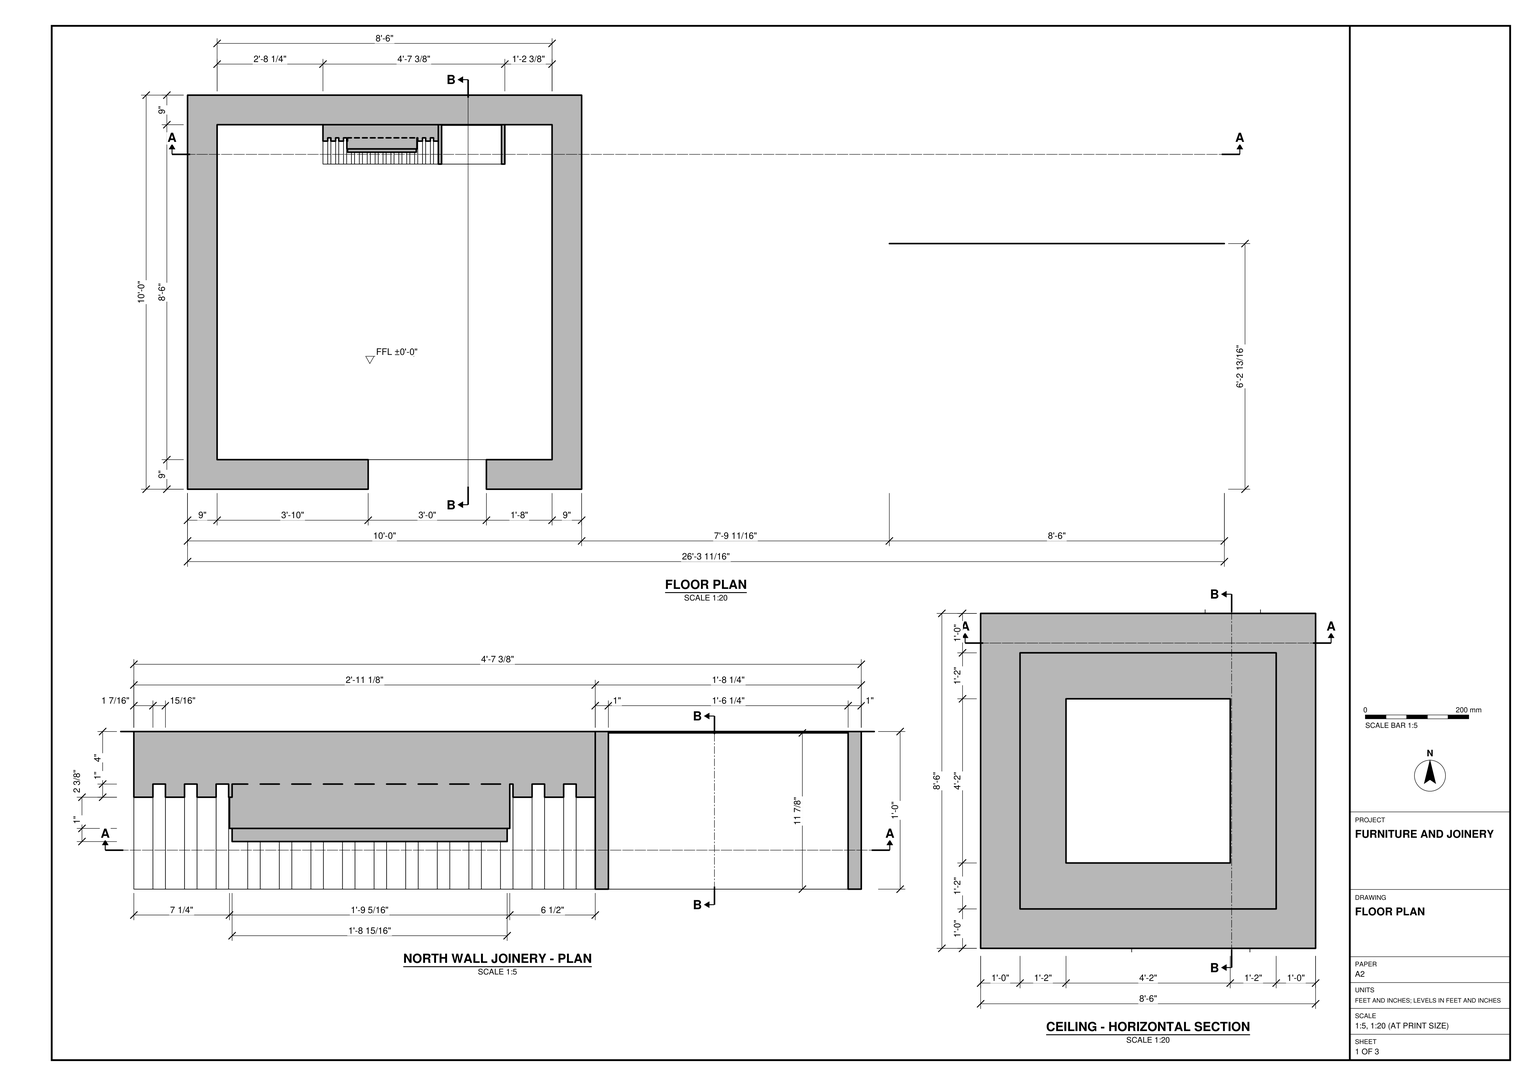
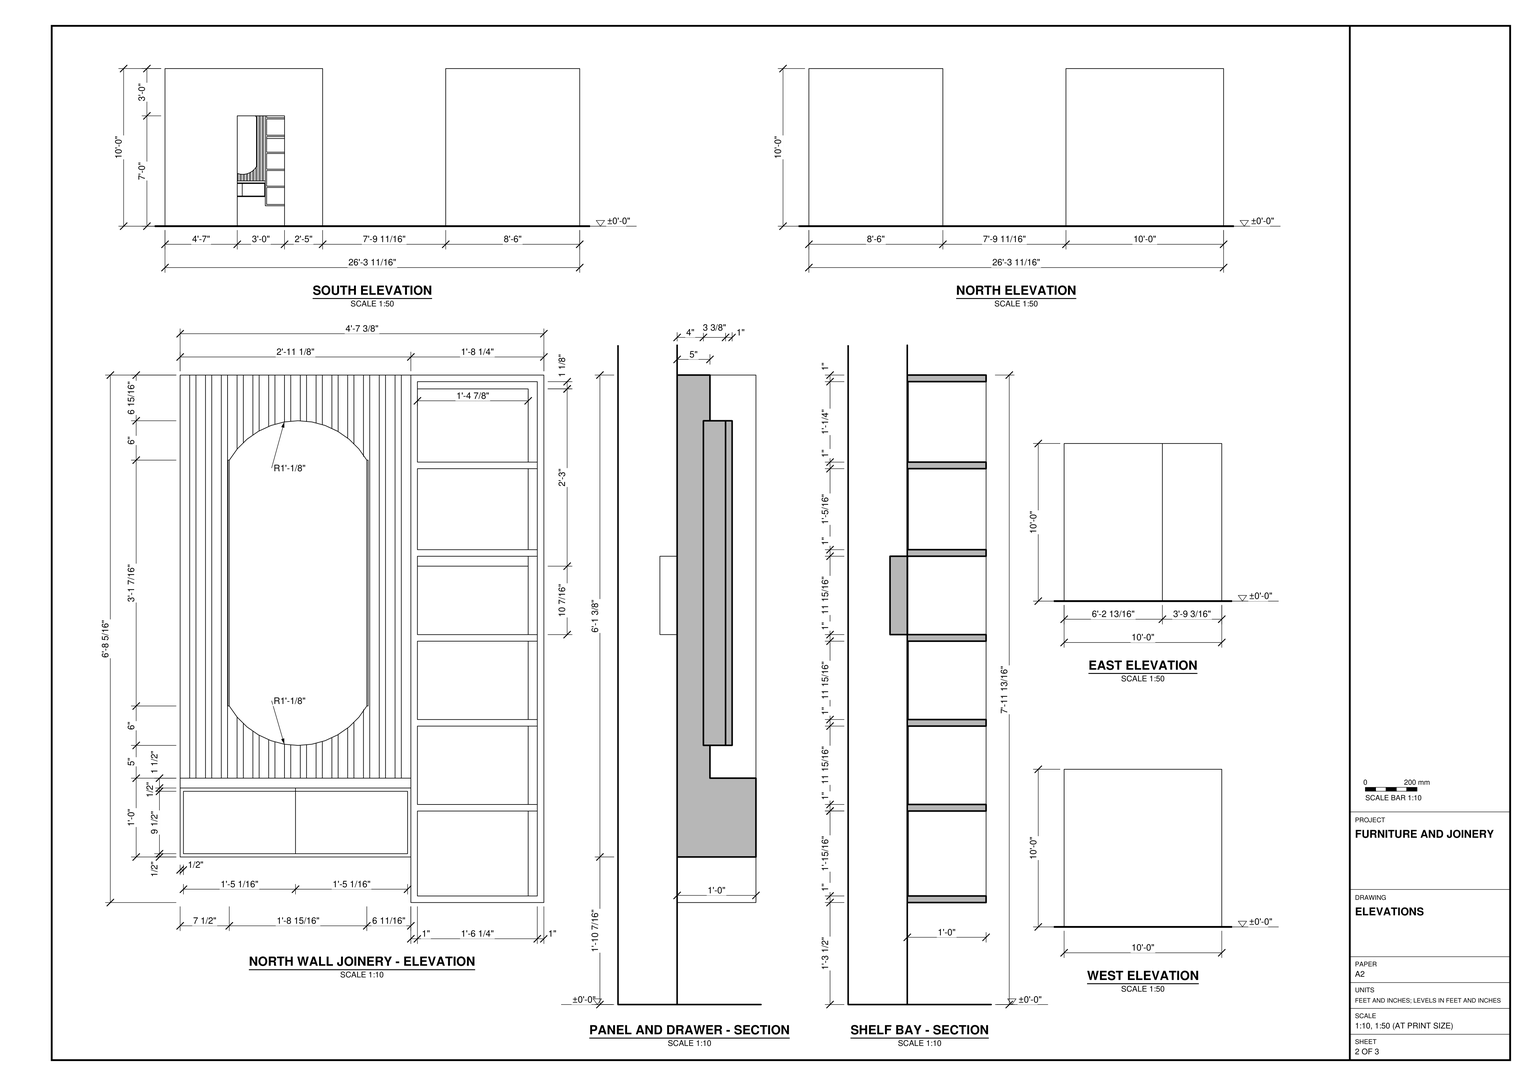
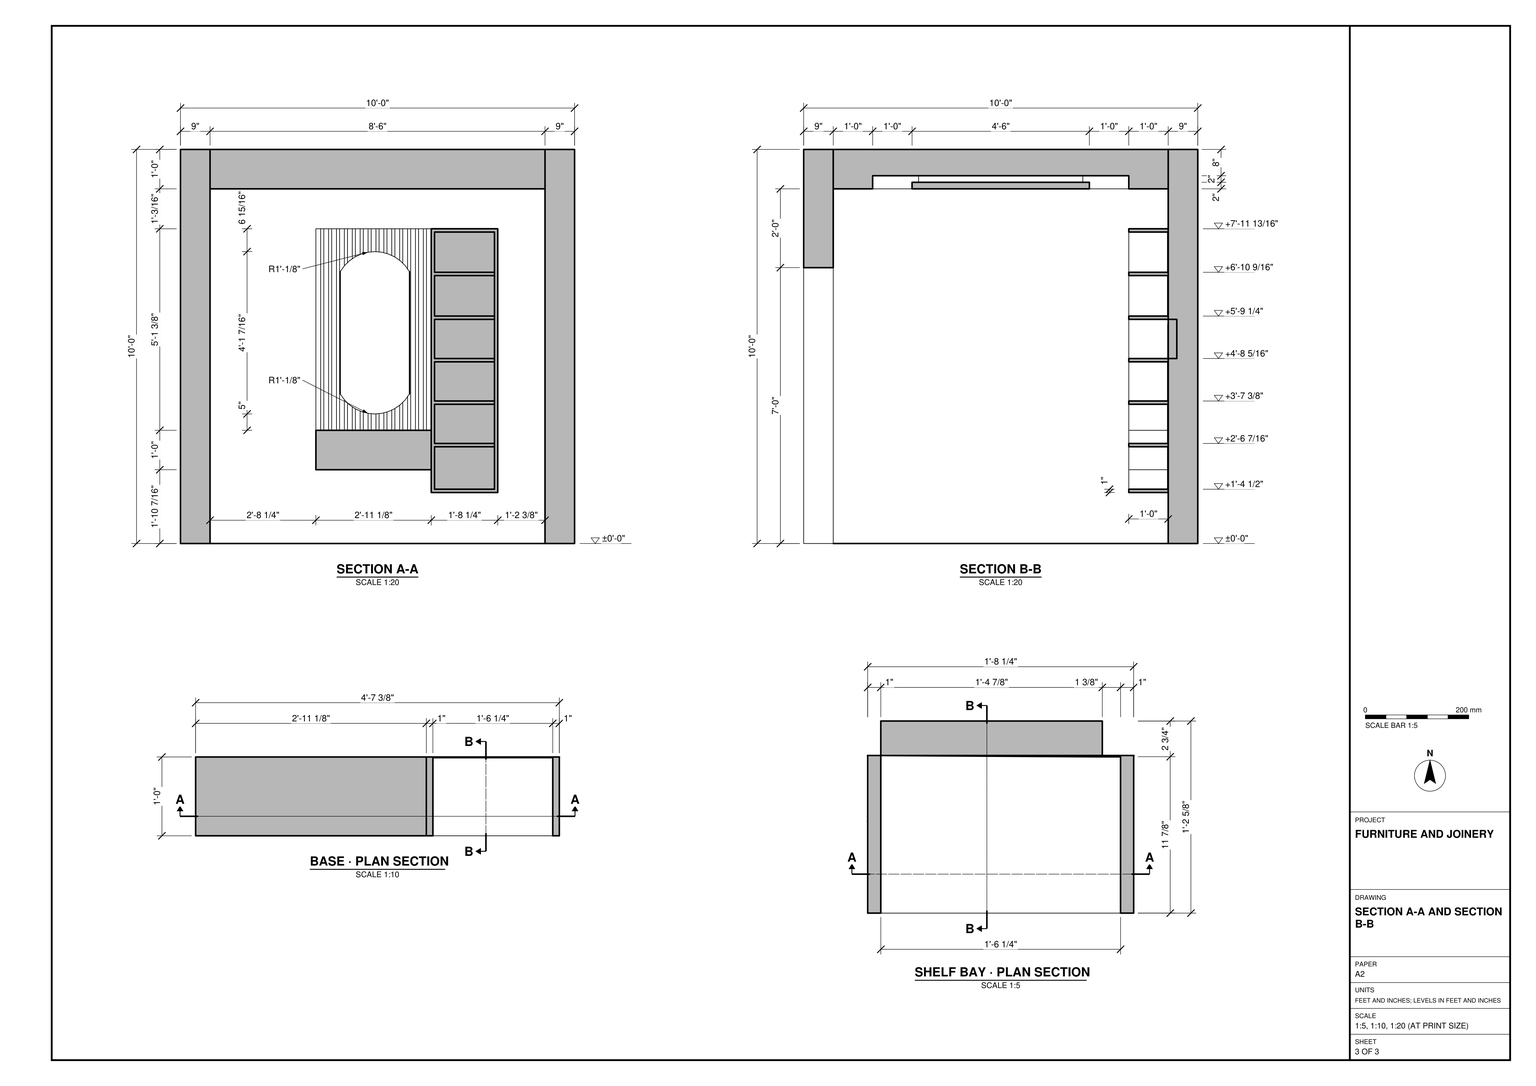
Build the room and its fitted joinery in SketchUp from task_files/diagram_01.pdf. Work in feet and inches. The overall model is 26'-3 11/16" along X, 10'-0" along Y and 10'-0" high, with a single finished floor level at ±0'-0". The room itself is 10'-0" square externally. The remaining X extent includes the gap and the separate upright surface shown east of the room; use the floor plan to locate that surface and the elevations to set its height.

Build the 9" perimeter walls and leave the offset doorway in the south wall, with the wall continuing above the opening. Form the stepped ceiling using the ceiling horizontal section for the square outlines and section B-B for their depths.

Fit the joinery against the inside of the north wall. Use the detailed elevation to lay out the wide, vertically slatted mirror panel on the left, the suspended drawer unit beneath it and the narrower open shelf bay on the right. Model the mirror with straight sides and curved ends. Align the tops of the two bays, but extend the shelving below the drawer unit as shown. Use the detailed sections to set the projections, shelf thicknesses and mounting heights.

Keep the shell elements and each joinery or furniture piece in separate groups or components, and use components for repeated parts. Any decor or loose items shown may use suitable library components. Save one SketchUp model as output_files/room_and_its_north_wall_mirror_and_shelf_unit.skp.

# SketchUp Ruby script. Lengths in inches.
U = 1.inch
M = Sketchup.active_model
def pt(a) = Geom::Point3d.new(a.map { |v| v * U })
def face(e, loops, mat)
  f = e.add_face(loops[0].map { |a| pt(a) })
  loops[1..].each { |l| e.add_face(l.map { |a| pt(a) }).erase! }
  f.material = f.back_material = mat if mat
  f
end
# faces: each face lists its corners as indices into pts; further lists are holes
def faces(e, pts, list, mat = nil) = list.each { |f| face(e, (f[0].is_a?(Array) ? f : [f]).map { |l| l.map { |i| pts[i] } }, mat) }
# xy, xz, yz: faces in a plane at the given z, y or x. An outline is a flat list of corners, or four numbers for a rectangle; further outlines are holes
def ring(l) = l.size == 4 ? [[l[0], l[1]], [l[2], l[1]], [l[2], l[3]], [l[0], l[3]]] : l.each_slice(2).to_a
def flat(e, list, mat, &to3) = list.each { |f| face(e, (f[0].is_a?(Array) ? f : [f]).map { |l| ring(l).map { |u, v| to3.(u, v) } }, mat) }
def xy(e, z, list, mat = nil) = flat(e, list, mat) { |x, y| [x, y, z] }
def xz(e, y, list, mat = nil) = flat(e, list, mat) { |x, z| [x, y, z] }
def yz(e, x, list, mat = nil) = flat(e, list, mat) { |y, z| [x, y, z] }
def lines(e, pts, list) = list.each { |a, b| e.add_line(pt(pts[a]), pt(pts[b])) }
# prism: a flat outline (further loops are holes) pulled along v
def prism(e, loops, v, mat = nil)
  f = face(e, loops, mat); d = Geom::Vector3d.new(v.map { |x| x * U })
  f.pushpull(f.normal.samedirection?(d) ? d.length : -d.length)
end
def box(e, o, s, mat = nil) = prism(e, [[o, [o[0] + s[0], o[1], o[2]], [o[0] + s[0], o[1] + s[1], o[2]], [o[0], o[1] + s[1], o[2]]]], [0, 0, s[2]], mat)
def at(x, y, z, deg = 0) = Geom::Transformation.translation(pt([x, y, z])) * Geom::Transformation.rotation(ORIGIN, Z_AXIS, deg.degrees)
def axes(o, x, y, z) = Geom::Transformation.new([*x, 0, *y, 0, *z, 0, *pt(o).to_a, 1])
def part(name) = M.definitions.add(name)
# library, detail: a bought-in or finely detailed component or shape, given as its bounding box
def library(name, o, s) = part(name).tap { |d| box(d.entities, o, s) }
def detail(e, o, s) = box(e.add_group.entities, o, s)
def put(e, d, t, mat = nil) = e.add_instance(d, t).tap { |i| i.material = mat if mat }
def group(e, t, mat = nil) = e.add_group.tap { |g| g.transformation = t; g.material = mat if mat }.entities
root = M.entities
M.materials.add("[Color A01]").color = [255, 204, 204]
M.materials.add("[Color A01]1").color = [255, 204, 204]
M.materials.add("[Color A01]2").color = [255, 247, 239]
M.materials.add("[Color M01]").color = [226, 226, 226]
M.materials.add("[Color M05]").color = [114, 114, 114]
M.materials.add("[Mirror 01]").color = [185, 185, 185]
M.materials.add("[Wood Bamboo]").color = [177, 105, 43]
M.materials.add("[Wood Veneer 01]").color = [120, 70, 37]
c1 = part("Component\#1")
xz(c1.entities,0,[[0,0,102,120]])
xy(root,0,[[0,0,0,120,120,120,120,0,91,0,91,9,111,9,111,111,9,111,9,9,55,9,55,0],[9,9,111,111]])
xy(root,84,[[55,0,91,9]])
xy(root,120,[[[0,0,120,120],[9,9,111,111]]])
xz(root,0,[[0,0,55,0,55,84,91,84,91,0,120,0,120,120,0,120]])
xz(root,9,[[9,0,9,120,111,120,111,0,91,0,91,84,55,84,55,0]])
xz(root,111,[[9,0,111,120]])
xz(root,120,[[0,0,120,120]])
yz(root,0,[[0,0,120,120]])
yz(root,9,[[9,0,111,120]])
yz(root,55,[[0,0,9,84]])
yz(root,76.36,[[99,34.47,106,95.84]],"[Wood Bamboo]")
yz(root,91,[[0,0,9,84]])
yz(root,111,[[9,0,111,120]])
yz(root,120,[[0,0,120,120]])
g1 = group(root,at(213.7,74.8,0))
xy(g1,15.53,[[-137.34,24.2,-117.09,36.2]],"[Wood Veneer 01]")
xy(g1,16.53,[[-119.48,36.1,-118.09,36.2]],"[Color A01]1")
xy(g1,16.53,[[-136.34,24.2,-118.09,36.1],[-136.34,36.1,-119.48,36.2]],"[Wood Veneer 01]")
xy(g1,22.47,[[-172.47,24.2,-137.34,36.2]])
xy(g1,29.46,[[-119.48,36.1,-118.09,36.2]],"[Color A01]1")
xy(g1,29.46,[[-136.34,24.2,-118.09,36.1],[-136.34,36.1,-119.48,36.2]],"[Wood Veneer 01]")
xy(g1,30.46,[[-119.48,36.1,-118.09,36.2]],"[Color A01]1")
xy(g1,30.46,[[-136.34,24.2,-118.09,36.1],[-136.34,36.1,-119.48,36.2]],"[Wood Veneer 01]")
xy(g1,34.47,[[-172.47,24.2,-171.01,31.2],[-171.01,24.2,-170.06,32.2],[-170.06,24.2,-168.61,31.2],[-168.61,24.2,-167.65,32.2],[-167.65,24.2,-166.2,31.2],
  [-166.2,24.2,-165.25,32.2],[-165.25,24.2,-163.8,31.2],[-163.8,24.2,-162.84,32.2],[-162.84,24.2,-161.39,31.2],[-161.39,24.2,-160.44,32.2],
  [-160.44,24.2,-158.99,31.2],[-158.99,24.2,-158.03,32.2],[-158.03,24.2,-156.58,31.2],[-156.58,24.2,-155.63,32.2],[-155.63,24.2,-154.18,31.2],
  [-154.18,24.2,-153.22,32.2],[-153.22,24.2,-151.77,31.2],[-151.77,24.2,-150.82,32.2],[-150.82,24.2,-149.37,31.2],[-149.37,24.2,-148.41,32.2],
  [-148.41,24.2,-146.96,31.2],[-146.96,24.2,-146.01,32.2],[-146.01,24.2,-144.56,31.2],[-144.56,24.2,-143.6,32.2],[-143.6,24.2,-142.15,31.2],
  [-142.15,24.2,-141.2,32.2],[-141.2,24.2,-139.75,31.2],[-139.75,24.2,-138.79,32.2],[-138.79,24.2,-137.34,31.2]])
xy(g1,39.64,[[-156.61,31.2,-156.58,32.2]])
xy(g1,42.4,[[-119.48,36.1,-118.09,36.2]],"[Color A01]1")
xy(g1,42.4,[[-136.34,24.2,-118.09,36.1],[-136.34,36.1,-119.48,36.2]],"[Wood Veneer 01]")
xy(g1,43.4,[[-119.48,36.1,-118.09,36.2]],"[Color A01]1")
xy(g1,43.4,[[-136.34,24.2,-118.09,36.1],[-136.34,36.1,-119.48,36.2]],"[Wood Veneer 01]")
xy(g1,45.46,[[-165.19,28.83,-164.99,31.2],[-144.05,28.83,-143.85,32.2]],"[Color A01]")
xy(g1,55.33,[[-119.48,36.1,-118.09,36.2]],"[Color A01]1")
xy(g1,55.33,[[-136.34,24.2,-118.09,36.1],[-136.34,36.1,-119.48,36.2]],"[Wood Veneer 01]")
xy(g1,56.33,[[-119.48,36.1,-119.48,36.2,-136.34,36.2]])
xy(g1,56.33,[[-119.48,36.1,-118.09,36.2]],"[Color A01]1")
xy(g1,56.33,[[-136.34,24.2,-118.09,24.2,-118.09,36.1,-119.48,36.1,-136.34,36.2],[-136.34,36.2,-119.48,38.83]],"[Wood Veneer 01]")
xy(g1,68.26,[[-119.48,36.1,-118.09,36.2]],"[Color A01]1")
xy(g1,68.26,[[-136.34,24.2,-136.34,36.2,-119.48,36.2,-119.48,36.1,-118.09,36.1,-118.09,24.2],[-136.34,36.2,-119.48,38.83]],"[Wood Veneer 01]")
xy(g1,69.26,[[-119.48,36.1,-118.09,36.2]],"[Color A01]1")
xy(g1,69.26,[[-136.34,24.2,-118.09,36.1],[-136.34,36.1,-119.48,36.2]],"[Wood Veneer 01]")
xy(g1,81.59,[[-119.48,36.1,-118.09,36.2]],"[Color A01]1")
xy(g1,81.59,[[-136.34,24.2,-118.09,36.1],[-136.34,36.1,-119.48,36.2]],"[Wood Veneer 01]")
xy(g1,82.59,[[-119.48,36.1,-118.09,36.2]],"[Color A01]1")
xy(g1,82.59,[[-136.34,24.2,-118.09,36.1],[-136.34,36.1,-119.48,36.2]],"[Wood Veneer 01]")
xy(g1,82.89,[[-165.19,28.83,-164.99,31.2],[-144.05,28.83,-143.85,32.2]],"[Color A01]")
xy(g1,88.71,[[-156.61,31.2,-156.58,32.2]])
xy(g1,94.84,[[-136.34,36.1,-118.09,36.2]],"[Color A01]1")
xy(g1,94.84,[[-136.34,24.2,-118.09,36.1]],"[Wood Veneer 01]")
xy(g1,95.84,[[-172.47,31.2,-171.01,31.2,-171.01,32.2,-170.06,32.2,-170.06,31.2,-168.61,31.2,-168.61,32.2,-167.65,32.2,-167.65,31.2,-166.2,31.2,-166.2,32.2,-165.25,32.2,-165.25,31.2,-163.8,31.2,-163.8,32.2,-162.84,32.2,-162.84,31.2,-161.39,31.2,-161.39,32.2,-160.44,32.2,-160.44,31.2,-158.99,31.2,-158.99,32.2,-158.03,32.2,-158.03,31.2,-156.58,31.2,-156.58,32.2,-155.63,32.2,-155.63,31.2,-154.18,31.2,-154.18,32.2,-153.22,32.2,-153.22,31.2,-151.77,31.2,-151.77,32.2,-150.82,32.2,-150.82,31.2,-149.37,31.2,-149.37,32.2,-148.41,32.2,-148.41,31.2,-146.96,31.2,-146.96,32.2,-146.01,32.2,-146.01,31.2,-144.56,31.2,-144.56,32.2,-143.6,32.2,-143.6,31.2,-142.15,31.2,-142.15,32.2,-141.2,32.2,-141.2,31.2,-139.75,31.2,-139.75,32.2,-138.79,32.2,-138.79,31.2,-137.34,31.2,-137.34,36.2,-172.47,36.2]])
xy(g1,95.84,[[-137.34,24.2,-117.09,36.2]],"[Wood Veneer 01]")
xz(g1,24.2,[[-172.47,22.47,-137.34,22.47,-137.34,32.97,-154.9,32.97,-154.9,32.47,-137.84,32.47,-137.84,22.97,-171.97,22.97,-171.97,32.47,-154.9,32.47,-154.9,32.97,-172.47,32.97],[-171.97,22.97,-154.9,32.47],[-154.9,22.97,-137.84,32.47]])
xz(g1,24.2,[[-172.47,32.97,-137.34,34.47]],"[Color M05]")
xz(g1,24.2,[[[-137.34,15.53,-117.09,95.84],[-136.34,16.53,-136.34,29.46,-118.09,29.46,-118.09,30.46,-136.34,30.46,-136.34,42.4,-118.09,42.4,-118.09,43.4,-136.34,43.4,-136.34,55.33,-118.09,55.33,-118.09,56.33,-136.34,56.33,-136.34,68.26,-118.09,68.26,-118.09,69.26,-136.34,69.26,-136.34,81.59,-118.09,81.59,-118.09,82.59,-136.34,82.59,-136.34,94.84,-118.09,94.84,-118.09,16.53]]],"[Wood Veneer 01]")
xz(g1,27.83,[[-154.52,39.46,-152.42,39.64,-150.39,40.18,-148.48,41.0625,-146.76,42.26,-145.26,43.74,-144.05,45.46,-144.05,82.89,-145.26,84.61,-146.76,86.09,-148.48,87.29,-150.39,88.17,-152.42,88.71,-154.52,88.89,-156.61,88.71,-158.64,88.17,-160.55,87.29,-162.28,86.09,-163.77,84.61,-164.99,82.89,-164.99,45.46,-163.77,43.74,-162.28,42.26,-160.55,41.0625,-158.64,40.18,-156.61,39.64]],"[Mirror 01]")
xz(g1,28.83,[[-154.52,39.46,-156.61,39.64,-158.64,40.18,-160.55,41.0625,-162.28,42.26,-163.77,43.74,-164.99,45.46,-164.99,82.89,-163.77,84.61,-162.28,86.09,-160.55,87.29,-158.64,88.17,-156.61,88.71,-154.52,88.89,-152.42,88.71,-150.39,88.17,-148.48,87.29,-146.76,86.09,-145.26,84.61,-144.05,82.89,-144.05,45.46,-145.26,43.74,-146.76,42.26,-148.48,41.0625,-150.39,40.18,-152.42,39.64]])
xz(g1,28.83,[[-165.19,45.46,-164.99,82.89],[-144.05,45.46,-143.85,82.89]],"[Color A01]")
xz(g1,31.2,[[-172.47,34.47,-171.01,95.84],[-170.06,34.47,-168.61,95.84],[-167.65,34.47,-166.2,95.84],[-165.25,34.47,-163.8,34.47,-163.8,43.78,-164.99,45.46,-165.19,45.46,-165.19,82.89,-164.99,82.89,-163.8,84.57,-163.8,95.84,-165.25,95.84],[-162.84,34.47,-161.39,34.47,-161.39,41.65,-162.28,42.26,-162.84,42.83],
  [-160.44,34.47,-158.99,34.47,-158.99,40.34,-160.44,41.01],[-158.03,34.47,-156.58,34.47,-156.58,39.64,-156.61,39.64,-158.03,40.02],[-155.63,34.47,-154.18,34.47,-154.18,39.49,-154.52,39.46,-155.63,39.55],[-153.22,34.47,-151.77,34.47,-151.77,39.8125,-152.42,39.64,-153.22,39.57],[-150.82,34.47,-149.37,34.47,-149.37,40.65,-150.39,40.18,-150.82,40.07],
  [-148.41,34.47,-146.96,34.47,-146.96,42.12,-148.41,41.11],[-146.01,34.47,-144.56,34.47,-144.56,44.74,-145.26,43.74,-146.01,43],[-143.6,34.47,-142.15,95.84],[-141.2,34.47,-139.75,95.84],[-138.79,34.47,-137.34,95.84],
  [-144.56,83.61,-144.56,95.84,-146.01,95.84,-146.01,85.35,-145.26,84.61],[-162.84,85.52,-162.28,86.09,-161.39,86.7,-161.39,95.84,-162.84,95.84],[-146.96,86.23,-146.96,95.84,-148.41,95.84,-148.41,87.24],[-160.44,87.34,-158.99,88.01,-158.99,95.84,-160.44,95.84],[-149.37,87.7,-149.37,95.84,-150.82,95.84,-150.82,88.28,-150.39,88.17],
  [-158.03,88.33,-156.61,88.71,-156.58,88.71,-156.58,95.84,-158.03,95.84],[-151.77,88.54,-151.77,95.84,-153.22,95.84,-153.22,88.78,-152.42,88.71],[-155.63,88.8,-154.52,88.89,-154.18,88.86,-154.18,95.84,-155.63,95.84]])
xz(g1,31.2,[[-165.19,45.46,-164.99,82.89]],"[Color A01]")
xz(g1,32.2,[[-171.01,34.47,-170.06,95.84],[-168.61,34.47,-167.65,95.84],[-166.2,34.47,-165.25,95.84],[-163.8,34.47,-162.84,34.47,-162.84,42.83,-163.77,43.74,-163.8,43.78],[-161.39,34.47,-160.44,34.47,-160.44,41.01,-160.55,41.0625,-161.39,41.65],
  [-158.99,34.47,-158.03,34.47,-158.03,40.02,-158.64,40.18,-158.99,40.34],[-156.58,34.47,-155.63,34.47,-155.63,39.55,-156.58,39.64],[-154.18,34.47,-153.22,34.47,-153.22,39.57,-154.18,39.49],[-151.77,34.47,-150.82,34.47,-150.82,40.07,-151.77,39.8125],[-149.37,34.47,-148.41,34.47,-148.41,41.11,-148.48,41.0625,-149.37,40.65],
  [-146.96,34.47,-146.01,34.47,-146.01,43,-146.76,42.26,-146.96,42.12],[-144.56,34.47,-143.6,34.47,-143.6,95.84,-144.56,95.84,-144.56,83.61,-144.05,82.89,-143.85,82.89,-143.85,45.46,-144.05,45.46,-144.56,44.74],[-142.15,34.47,-141.2,95.84],[-139.75,34.47,-138.79,95.84],[-154.52,39.46,-154.18,39.49,-154.18,88.86,-154.52,88.89,-155.63,88.8,-155.63,39.55],
  [-153.22,39.57,-152.42,39.64,-151.77,39.8125,-151.77,88.54,-152.42,88.71,-153.22,88.78],[-156.61,39.64,-156.58,39.64,-156.58,88.71,-156.61,88.71,-158.03,88.33,-158.03,40.02],[-150.82,40.07,-150.39,40.18,-149.37,40.65,-149.37,87.7,-150.39,88.17,-150.82,88.28],[-158.99,40.34,-158.99,88.01,-160.44,87.34,-160.44,41.01],[-148.41,41.11,-146.96,42.12,-146.96,86.23,-148.41,87.24],
  [-161.39,41.65,-161.39,86.7,-162.28,86.09,-162.84,85.52,-162.84,42.83,-162.28,42.26],[-146.01,43,-145.26,43.74,-144.56,44.74,-144.56,83.61,-145.26,84.61,-146.01,85.35],[-163.8,43.78,-163.8,84.57,-164.99,82.89,-164.99,45.46],[-163.8,84.57,-163.77,84.61,-162.84,85.52,-162.84,95.84,-163.8,95.84],[-146.01,85.35,-146.01,95.84,-146.96,95.84,-146.96,86.23,-146.76,86.09],
  [-161.39,86.7,-160.55,87.29,-160.44,87.34,-160.44,95.84,-161.39,95.84],[-148.41,87.24,-148.41,95.84,-149.37,95.84,-149.37,87.7,-148.48,87.29],[-158.99,88.01,-158.64,88.17,-158.03,88.33,-158.03,95.84,-158.99,95.84],[-150.82,88.28,-150.82,95.84,-151.77,95.84,-151.77,88.54],[-156.58,88.71,-155.63,88.8,-155.63,95.84,-156.58,95.84],
  [-153.22,88.78,-153.22,95.84,-154.18,95.84,-154.18,88.86]])
xz(g1,36.1,[[-119.48,16.53,-118.09,29.46],[-119.48,30.46,-118.09,42.4],[-119.48,43.4,-118.09,55.33],[-119.48,56.33,-118.09,68.26],[-119.48,69.26,-118.09,81.59],
  [-119.48,82.59,-118.09,82.59,-118.09,94.84,-136.34,94.84,-136.34,93.74,-119.48,93.74]],"[Color A01]1")
xz(g1,36.1,[[-136.34,16.53,-119.48,29.46],[-136.34,30.46,-119.48,42.4],[-136.34,43.4,-119.48,55.33],[-136.34,69.26,-119.48,81.59],[-136.34,82.59,-119.48,93.74]],"[Wood Veneer 01]")
xz(g1,36.2,[[[-137.34,15.53,-117.09,95.84],[-136.34,16.53,-118.09,16.53,-118.09,94.84,-136.34,94.84,-136.34,82.59,-118.09,82.59,-118.09,81.59,-136.34,81.59,-136.34,69.26,-118.09,69.26,-118.09,68.26,-136.34,68.26,-136.34,56.33,-118.09,56.33,-118.09,55.33,-136.34,55.33,-136.34,43.4,-118.09,43.4,-118.09,42.4,-136.34,42.4,-136.34,30.46,-118.09,30.46,-118.09,29.46,-136.34,29.46]],[-172.47,22.47,-137.34,95.84]])
xz(g1,38.83,[[-136.34,56.33,-119.48,68.26]],"[Wood Veneer 01]")
yz(g1,-172.47,[[31.2,34.47,36.2,95.84]])
yz(g1,-172.47,[[24.2,22.47,36.2,34.47]],"[Color M05]")
yz(g1,-171.01,[[31.2,34.47,32.2,95.84]])
yz(g1,-170.06,[[31.2,34.47,32.2,95.84]])
yz(g1,-168.61,[[31.2,34.47,32.2,95.84]])
yz(g1,-167.65,[[31.2,34.47,32.2,95.84]])
yz(g1,-166.2,[[31.2,34.47,32.2,95.84]])
yz(g1,-165.25,[[31.2,34.47,32.2,95.84]])
yz(g1,-165.19,[[28.83,45.46,31.2,82.89]],"[Color A01]")
yz(g1,-164.99,[[27.83,45.46,28.83,82.89],[31.2,45.46,32.2,82.89]])
yz(g1,-163.8,[[31.2,34.47,32.2,43.78],[31.2,84.57,32.2,95.84]])
yz(g1,-162.84,[[31.2,34.47,32.2,42.83],[31.2,85.52,32.2,95.84]])
yz(g1,-161.39,[[31.2,34.47,32.2,41.65],[31.2,86.7,32.2,95.84]])
yz(g1,-160.44,[[31.2,34.47,32.2,41.01],[31.2,87.34,32.2,95.84]])
yz(g1,-158.99,[[31.2,34.47,32.2,40.34],[31.2,88.01,32.2,95.84]])
yz(g1,-158.03,[[31.2,34.47,32.2,40.02],[31.2,88.33,32.2,95.84]])
yz(g1,-156.58,[[31.2,34.47,32.2,39.64],[31.2,88.71,32.2,95.84]])
yz(g1,-155.63,[[31.2,34.47,32.2,39.55],[31.2,88.8,32.2,95.84]])
yz(g1,-154.18,[[31.2,34.47,32.2,39.49],[31.2,88.86,32.2,95.84]])
yz(g1,-153.22,[[31.2,34.47,32.2,39.57],[31.2,88.78,32.2,95.84]])
yz(g1,-151.77,[[31.2,34.47,32.2,39.8125],[31.2,88.54,32.2,95.84]])
yz(g1,-150.82,[[31.2,34.47,32.2,40.07],[31.2,88.28,32.2,95.84]])
yz(g1,-149.37,[[31.2,34.47,32.2,40.65],[31.2,87.7,32.2,95.84]])
yz(g1,-148.41,[[31.2,34.47,32.2,41.11],[31.2,87.24,32.2,95.84]])
yz(g1,-146.96,[[31.2,34.47,32.2,42.12],[31.2,86.23,32.2,95.84]])
yz(g1,-146.01,[[31.2,34.47,32.2,43],[31.2,85.35,32.2,95.84]])
yz(g1,-144.56,[[31.2,34.47,32.2,44.74],[31.2,83.61,32.2,95.84]])
yz(g1,-144.05,[[27.83,45.46,28.83,82.89]])
yz(g1,-143.85,[[28.83,45.46,32.2,82.89]],"[Color A01]")
yz(g1,-143.6,[[31.2,34.47,32.2,95.84]])
yz(g1,-142.15,[[31.2,34.47,32.2,95.84]])
yz(g1,-141.2,[[31.2,34.47,32.2,95.84]])
yz(g1,-139.75,[[31.2,34.47,32.2,95.84]])
yz(g1,-138.79,[[31.2,34.47,32.2,95.84]])
yz(g1,-137.34,[[24.2,22.47,36.2,34.47],[24.2,34.47,31.2,95.84],[31.2,34.47,36.2,95.84]])
yz(g1,-137.34,[[24.2,15.53,36.2,22.47]],"[Wood Veneer 01]")
yz(g1,-136.34,[[36.1,93.74,36.2,94.84]],"[Color A01]1")
yz(g1,-136.34,[[24.2,16.53,36.1,22.47],[36.1,16.53,36.2,22.47],[24.2,22.47,36.1,29.46],[36.1,22.47,36.2,29.46],[24.2,30.46,36.1,34.47],
  [36.1,30.46,36.2,34.47],[24.2,34.47,36.1,42.4],[36.1,34.47,36.2,42.4],[24.2,43.4,36.1,55.33],[36.1,43.4,36.2,55.33],
  [24.2,56.33,36.2,68.26],[36.2,56.33,38.83,68.26],[24.2,69.26,36.1,81.59],[36.1,69.26,36.2,81.59],[24.2,82.59,36.1,94.84],
  [36.1,82.59,36.2,93.74]],"[Wood Veneer 01]")
yz(g1,-119.48,[[36.1,56.33,38.83,68.26]],"[Color A01]1")
yz(g1,-118.09,[[24.2,29.46,36.2,30.46],[24.2,42.4,36.2,43.4],[24.2,55.33,36.2,56.33],[24.2,68.26,36.2,69.26],[24.2,81.59,36.2,82.59]])
yz(g1,-118.09,[[36.1,16.53,36.2,29.46],[36.1,30.46,36.2,42.4],[36.1,43.4,36.2,55.33],[36.1,56.33,36.2,68.26],[36.1,69.26,36.2,81.59],
  [36.1,82.59,36.2,94.84]],"[Color A01]1")
yz(g1,-118.09,[[24.2,16.53,36.1,29.46],[24.2,30.46,36.1,42.4],[24.2,43.4,36.1,55.33],[24.2,56.33,36.1,68.26],[24.2,69.26,36.1,81.59],
  [24.2,82.59,36.1,94.84]],"[Wood Veneer 01]")
yz(g1,-117.09,[[24.2,15.53,36.2,95.84]],"[Wood Veneer 01]")
p = [[-156.61,28.83,39.64],[-154.52,28.83,39.46],[-154.52,27.83,39.46],[-156.61,27.83,39.64],[-152.42,28.83,39.64],[-152.42,27.83,39.64],
  [-156.61,31.2,39.64],[-156.58,31.2,39.64],[-156.58,32.2,39.64],[-155.63,32.2,39.55],[-155.63,31.2,39.55],[-154.52,31.2,39.46],
  [-154.18,31.2,39.49],[-154.18,32.2,39.49],[-153.22,32.2,39.57],[-153.22,31.2,39.57],[-152.42,31.2,39.64],[-154.52,32.2,39.46],
  [-158.64,28.83,40.18],[-158.64,27.83,40.18],[-150.39,28.83,40.18],[-150.39,27.83,40.18],[-158.64,32.2,40.18],[-158.03,32.2,40.02],
  [-158.03,31.2,40.02],[-151.77,31.2,39.8125],[-151.77,32.2,39.8125],[-150.82,32.2,40.07],[-150.82,31.2,40.07],[-150.39,31.2,40.18],
  [-156.61,32.2,39.64],[-152.42,32.2,39.64],[-150.39,32.2,40.18],[-160.55,28.83,41.0625],[-160.55,27.83,41.0625],[-148.48,28.83,41.0625],
  [-148.48,27.83,41.0625],[-160.55,32.2,41.0625],[-160.44,32.2,41.01],[-160.44,31.2,41.01],[-158.99,31.2,40.34],[-158.99,32.2,40.34],
  [-149.37,31.2,40.65],[-149.37,32.2,40.65],[-148.48,32.2,41.0625],[-162.28,28.83,42.26],[-162.28,27.83,42.26],[-146.76,28.83,42.26],
  [-146.76,27.83,42.26],[-162.28,31.2,42.26],[-161.39,31.2,41.65],[-161.39,32.2,41.65],[-148.41,32.2,41.11],[-148.41,31.2,41.11],
  [-146.96,31.2,42.12],[-146.96,32.2,42.12],[-146.76,32.2,42.26],[-162.28,32.2,42.26],[-163.77,28.83,43.74],[-163.77,27.83,43.74],
  [-145.26,28.83,43.74],[-145.26,27.83,43.74],[-163.77,32.2,43.74],[-162.84,32.2,42.83],[-162.84,31.2,42.83],[-146.01,32.2,43],
  [-146.01,31.2,43],[-145.26,31.2,43.74],[-145.26,32.2,43.74],[-164.99,28.83,45.46],[-164.99,27.83,45.46],[-144.05,28.83,45.46],
  [-144.05,27.83,45.46],[-164.99,31.2,45.46],[-163.8,31.2,43.78],[-163.8,32.2,43.78],[-144.56,31.2,44.74],[-144.56,32.2,44.74],
  [-144.05,32.2,45.46],[-164.99,32.2,45.46],[-119.48,36.1,56.33],[-136.34,36.2,56.33],[-136.34,36.2,66.75],[-119.48,36.1,66.75],
  [-163.77,28.83,84.61],[-164.99,28.83,82.89],[-164.99,27.83,82.89],[-163.77,27.83,84.61],[-144.05,28.83,82.89],[-145.26,28.83,84.61],
  [-145.26,27.83,84.61],[-144.05,27.83,82.89],[-163.77,32.2,84.61],[-163.8,32.2,84.57],[-163.8,31.2,84.57],[-164.99,31.2,82.89],
  [-144.05,32.2,82.89],[-144.56,32.2,83.61],[-144.56,31.2,83.61],[-145.26,31.2,84.61],[-164.99,32.2,82.89],[-145.26,32.2,84.61],
  [-162.28,28.83,86.09],[-162.28,27.83,86.09],[-146.76,28.83,86.09],[-146.76,27.83,86.09],[-162.84,32.2,85.52],[-162.28,31.2,86.09],
  [-162.84,31.2,85.52],[-146.01,32.2,85.35],[-146.76,32.2,86.09],[-146.01,31.2,85.35],[-162.28,32.2,86.09],[-160.55,28.83,87.29],
  [-160.55,27.83,87.29],[-148.48,28.83,87.29],[-148.48,27.83,87.29],[-160.55,32.2,87.29],[-161.39,32.2,86.7],[-161.39,31.2,86.7],
  [-148.41,32.2,87.24],[-148.48,32.2,87.29],[-146.96,32.2,86.23],[-146.96,31.2,86.23],[-148.41,31.2,87.24],[-158.64,28.83,88.17],
  [-158.64,27.83,88.17],[-150.39,28.83,88.17],[-150.39,27.83,88.17],[-160.44,32.2,87.34],[-158.64,32.2,88.17],[-158.99,32.2,88.01],
  [-158.99,31.2,88.01],[-160.44,31.2,87.34],[-149.37,32.2,87.7],[-149.37,31.2,87.7],[-150.39,31.2,88.17],[-150.39,32.2,88.17],
  [-156.61,28.83,88.71],[-156.61,27.83,88.71],[-152.42,28.83,88.71],[-152.42,27.83,88.71],[-158.03,32.2,88.33],[-156.61,31.2,88.71],
  [-158.03,31.2,88.33],[-150.82,32.2,88.28],[-151.77,32.2,88.54],[-151.77,31.2,88.54],[-152.42,31.2,88.71],[-150.82,31.2,88.28],
  [-156.61,32.2,88.71],[-152.42,32.2,88.71],[-154.52,28.83,88.89],[-154.52,27.83,88.89],[-155.63,32.2,88.8],[-156.58,32.2,88.71],
  [-156.58,31.2,88.71],[-154.52,31.2,88.89],[-155.63,31.2,88.8],[-153.22,32.2,88.78],[-154.18,32.2,88.86],[-154.18,31.2,88.86],
  [-153.22,31.2,88.78],[-154.52,32.2,88.89]]
faces(g1,p,[[0,1,2,3],[1,4,5,2],[9,17,11,10],[17,13,12,11],[18,0,3,19],[4,20,21,5],[23,30,6,24],[14,31,16,15],
  [31,26,25,16],[27,32,29,28],[33,18,19,34],[20,35,36,21],[32,43,42,29],[38,41,40,39],[45,33,34,46],[35,47,48,36],
  [52,55,54,53],[57,51,50,49],[58,45,46,59],[47,60,61,48],[63,57,49,64],[65,68,67,66],[69,58,59,70],[60,71,72,61],
  [68,77,76,67],[79,75,74,73],[84,85,86,87],[88,89,90,91],[93,100,95,94],[97,101,99,98],[102,84,87,103],[89,104,105,90],
  [101,109,111,99],[112,106,108,107],[113,102,103,114],[104,115,116,105],[118,112,107,119],[122,120,124,123],[125,113,114,126],[115,127,128,116],
  [131,129,133,132],[134,137,136,135],[138,125,126,139],[127,140,141,128],[137,145,149,136],[150,142,144,143],[146,151,148,147],[152,138,139,153],
  [140,152,153,141],[151,159,162,148],[163,154,158,157],[160,163,157,161]])
faces(g1,p,[[0,6,7,8,9,10,11,1],[1,11,12,13,14,15,16,4],[22,23,24,6,0,18],[4,16,25,26,27,28,29,20],[37,38,39,40,41,22,18,33],[20,29,42,43,44,35],[45,49,50,51,37,33],[44,52,53,54,55,56,47,35],
  [62,63,64,49,45,58],[56,65,66,67,60,47],[69,73,74,75,62,58],[60,67,76,77,78,71],[92,93,94,95,85,84],[96,97,98,99,89,88],[106,92,84,102,107,108],[109,110,104,89,99,111],
  [117,118,119,107,102,113],[120,121,115,104,110,122,123,124],[129,117,113,125,130,131,132,133],[121,134,135,136,127,115],[142,130,125,138,143,144],[145,146,147,148,140,127,136,149],[154,155,156,143,138,152,157,158],[159,160,161,157,152,140,148,162]],"[Color A01]")
faces(g1,p,[[80,81,82,83]],"[Wood Veneer 01]")
put(g1,c1,at(0,0,0))
put(g1,c1,at(-204.7,36.2,0),"[Color M01]")
g2 = group(root,at(9,9,120))
xy(g2,-12,[[[0,0,102,102],[12,12,90,90]],[24,24,78,78]])
xy(g2,-10,[[24,24,78,26],[24,26,26,78],[26,26,76,76],[76,26,78,76],[26,76,78,78]])
xy(g2,-8,[[[12,12,90,90],[26,26,76,76]]])
xy(g2,0,[[0,0,102,102]])
xz(g2,0,[[0,-12,102,0]])
xz(g2,12,[[12,-12,90,-8]])
xz(g2,24,[[24,-12,78,-10]])
xz(g2,26,[[26,-10,76,-8]],"[Color A01]2")
xz(g2,76,[[26,-10,76,-8]],"[Color A01]2")
xz(g2,78,[[24,-12,78,-10]])
xz(g2,90,[[12,-12,90,-8]])
xz(g2,102,[[0,-12,102,0]])
yz(g2,0,[[0,-12,102,0]])
yz(g2,12,[[12,-12,90,-8]])
yz(g2,24,[[24,-12,78,-10]])
yz(g2,26,[[26,-10,76,-8]],"[Color A01]2")
yz(g2,76,[[26,-10,76,-8]],"[Color A01]2")
yz(g2,78,[[24,-12,78,-10]])
yz(g2,90,[[12,-12,90,-8]])
yz(g2,102,[[0,-12,102,0]])
